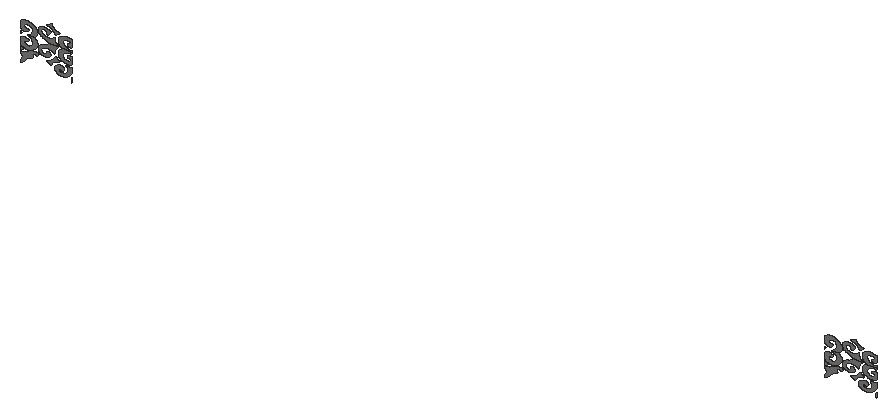
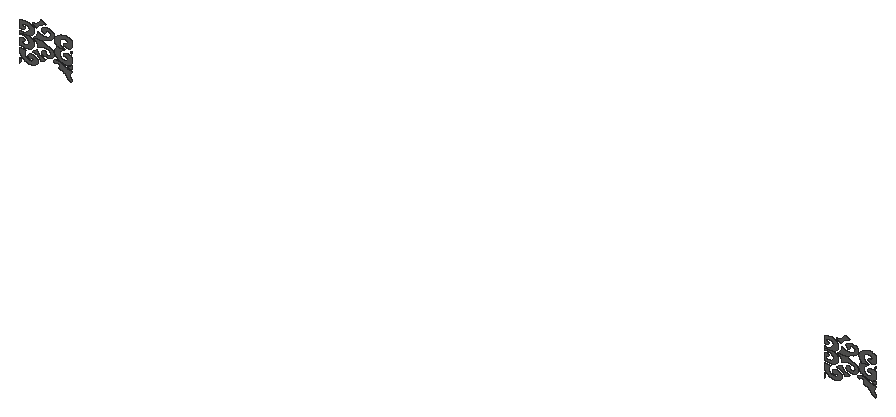
# SketchUp Ruby script. Lengths in inches.
U = 1.inch
M = Sketchup.active_model
def pt(a) = Geom::Point3d.new(a.map { |v| v * U })
def face(e, loops, mat)
  f = e.add_face(loops[0].map { |a| pt(a) })
  loops[1..].each { |l| e.add_face(l.map { |a| pt(a) }).erase! }
  f.material = f.back_material = mat if mat
  f
end
# faces: each face lists its corners as indices into pts; further lists are holes
def faces(e, pts, list, mat = nil) = list.each { |f| face(e, (f[0].is_a?(Array) ? f : [f]).map { |l| l.map { |i| pts[i] } }, mat) }
# xy, xz, yz: faces in a plane at the given z, y or x. An outline is a flat list of corners, or four numbers for a rectangle; further outlines are holes
def ring(l) = l.size == 4 ? [[l[0], l[1]], [l[2], l[1]], [l[2], l[3]], [l[0], l[3]]] : l.each_slice(2).to_a
def flat(e, list, mat, &to3) = list.each { |f| face(e, (f[0].is_a?(Array) ? f : [f]).map { |l| ring(l).map { |u, v| to3.(u, v) } }, mat) }
def xy(e, z, list, mat = nil) = flat(e, list, mat) { |x, y| [x, y, z] }
def xz(e, y, list, mat = nil) = flat(e, list, mat) { |x, z| [x, y, z] }
def yz(e, x, list, mat = nil) = flat(e, list, mat) { |y, z| [x, y, z] }
def lines(e, pts, list) = list.each { |a, b| e.add_line(pt(pts[a]), pt(pts[b])) }
# prism: a flat outline (further loops are holes) pulled along v
def prism(e, loops, v, mat = nil)
  f = face(e, loops, mat); d = Geom::Vector3d.new(v.map { |x| x * U })
  f.pushpull(f.normal.samedirection?(d) ? d.length : -d.length)
end
def box(e, o, s, mat = nil) = prism(e, [[o, [o[0] + s[0], o[1], o[2]], [o[0] + s[0], o[1] + s[1], o[2]], [o[0], o[1] + s[1], o[2]]]], [0, 0, s[2]], mat)
def at(x, y, z, deg = 0) = Geom::Transformation.translation(pt([x, y, z])) * Geom::Transformation.rotation(ORIGIN, Z_AXIS, deg.degrees)
def axes(o, x, y, z) = Geom::Transformation.new([*x, 0, *y, 0, *z, 0, *pt(o).to_a, 1])
def part(name) = M.definitions.add(name)
# library, detail: a bought-in or finely detailed component or shape, given as its bounding box
def library(name, o, s) = part(name).tap { |d| box(d.entities, o, s) }
def detail(e, o, s) = box(e.add_group.entities, o, s)
def put(e, d, t, mat = nil) = e.add_instance(d, t).tap { |i| i.material = mat if mat }
def group(e, t, mat = nil) = e.add_group.tap { |g| g.transformation = t; g.material = mat if mat }.entities
root = M.entities
M.materials.add("[0043_SaddleBrown]4").color = [124, 123, 122]
xz(root,589.17,[[449.07,580.05,448.85,580.56,448.66,581.07,448.52,581.59,448.42,582.11,448.35,582.63,448.33,583.15,448.35,583.68,448.42,584.2,448.52,584.72,448.66,585.24,448.85,585.75,449.07,586.26],[1699.7,580.05,1699.47,580.56,1699.29,581.07,1699.14,581.59,1699.04,582.11,1698.98,582.63,1698.96,583.15,1698.98,583.68,1699.04,584.2,1699.14,584.72,1699.29,585.24,1699.47,585.75,1699.7,586.26],[368.68,580.61,368.68,583.34,369.7,584.11,370.56,584.96,371.24,585.86,371.73,586.8125,372.03,587.79,372.13,588.78,372.03,589.78,371.73,590.76,371.24,591.71,370.56,592.61,369.7,593.46,368.68,594.23,368.68,595.13,369.97,595.29,371.24,595.5,372.49,595.74,373.72,596.03,374.93,596.35,376.1,596.71,377.24,597.11,378.35,597.55,379.42,598.02,380.44,598.53,381.42,599.0625,382.36,599.63,383.09,600.07,383.86,600.47,384.69,600.83,385.55,601.16,386.45,601.46,387.375,601.71,388.33,601.92,389.3125,602.08,390.31,602.21,391.32,602.28,392.33,602.32,393.35,602.31,394.16,602.23,394.92,602.03,395.6,601.74,396.15,601.36,396.54,600.91,396.76,600.43,396.8,599.92,396.65,599.42,396.32,598.95,395.83,598.54,395.21,598.21,394.48,597.98,394.37,598.49,394.05,598.96,393.54,599.37,392.875,599.68,392.1,599.88,391.27,599.95,390.45,599.88,389.67,599.68,389.01,599.37,388.5,598.96,388.18,598.49,388.07,597.98,388.03,597.57,388,597.17,387.99,596.76,388,596.36,388.03,595.95,388.07,595.55,388.14,595.15,388.22,594.74,388.3125,594.34,388.43,593.95,388.5625,593.55,388.71,593.15,387.25,592.79,385.84,592.36,384.48,591.86,383.2,591.3,381.99,590.67,380.87,589.99,379.84,589.26,378.91,588.48,378.08,587.65,377.37,586.79,376.76,585.89,376.27,584.97,375.75,584.54,375.2,584.125,374.64,583.72,374.05,583.32,373.44,582.94,372.81,582.57,372.17,582.21,371.51,581.86,370.82,581.53,370.125,581.21,369.41,580.9],[1619.31,580.61,1619.31,583.34,1620.33,584.11,1621.18,584.96,1621.86,585.86,1622.36,586.8125,1622.66,587.79,1622.76,588.78,1622.66,589.78,1622.36,590.76,1621.86,591.71,1621.18,592.61,1620.33,593.46,1619.31,594.23,1619.31,595.13,1620.59,595.29,1621.87,595.5,1623.12,595.74,1624.35,596.03,1625.55,596.35,1626.73,596.71,1627.87,597.11,1628.97,597.55,1630.04,598.02,1631.07,598.53,1632.05,599.0625,1632.98,599.63,1633.71,600.07,1634.49,600.47,1635.31,600.83,1636.17,601.16,1637.07,601.46,1638,601.71,1638.96,601.92,1639.9375,602.08,1640.93,602.21,1641.94,602.28,1642.95,602.32,1643.97,602.31,1644.79,602.23,1645.55,602.03,1646.22,601.74,1646.77,601.36,1647.17,600.91,1647.39,600.43,1647.43,599.92,1647.28,599.42,1646.95,598.95,1646.46,598.54,1645.83,598.21,1645.1,597.98,1644.99,598.49,1644.67,598.96,1644.16,599.37,1643.5,599.68,1642.73,599.88,1641.9,599.95,1641.07,599.88,1640.3,599.68,1639.63,599.37,1639.125,598.96,1638.81,598.49,1638.7,597.98,1638.65,597.57,1638.625,597.17,1638.62,596.76,1638.63,596.36,1638.65,595.95,1638.7,595.55,1638.76,595.15,1638.84,594.74,1638.9375,594.34,1639.05,593.95,1639.1875,593.55,1639.34,593.15,1637.875,592.79,1636.46,592.36,1635.11,591.86,1633.83,591.3,1632.62,590.67,1631.5,589.99,1630.47,589.26,1629.54,588.48,1628.71,587.65,1627.99,586.79,1627.39,585.89,1626.9,584.97,1626.375,584.54,1625.83,584.125,1625.26,583.72,1624.67,583.32,1624.07,582.94,1623.44,582.57,1622.79,582.21,1622.13,581.86,1621.45,581.53,1620.75,581.21,1620.04,580.9],[432.72,583.36,431.31,583.46,429.92,583.66,428.58,583.96,426.64,584.61,424.95,585.48,423.5625,586.54,422.53,587.74,421.9,589.04,421.68,590.39,421.9,591.74,422.53,593.04,423.5625,594.24,424.95,595.29,426.64,596.16,428.58,596.82,429.22,597.05,429.91,597.21,430.64,597.31,431.38,597.33,432.12,597.28,432.84,597.17,433.52,596.98,434.14,596.73,434.68,596.42,435.15,596.0625,435.51,595.66,435.77,595.23,436.13,594.85,436.41,594.45,436.58,594.02,436.66,593.58,436.63,593.14,436.51,592.7,436.29,592.28,435.97,591.89,435.5625,591.52,435.08,591.2,434.52,590.92,433.91,590.6875,433.55,590.8,433.21,590.93,432.88,591.07,432.57,591.23,432.28,591.4,432.01,591.58,431.76,591.78,431.54,591.98,431.33,592.19,431.15,592.41,431,592.64,430.87,592.87,430.1,592.59,429.4375,592.22,428.89,591.79,428.49,591.3,428.24,590.77,428.16,590.23,428.24,589.68,428.49,589.15,428.89,588.66,429.4375,588.23,430.1,587.86,430.87,587.58,431.8,587.56,432.73,587.58,433.66,587.64,434.58,587.75,435.48,587.9,436.36,588.09,437.22,588.32,438.04,588.58,438.84,588.89,439.59,589.23,440.3,589.6,440.96,590,441.54,590.79,442.01,591.6,442.36,592.43,442.58,593.28,442.68,594.14,442.65,595,442.5,595.85,442.22,596.7,441.82,597.52,441.3,598.32,440.67,599.09,439.92,599.82,440.68,599.65,441.47,599.53,442.26,599.46,443.07,599.42,443.87,599.43,444.67,599.48,445.47,599.57,446.24,599.7,447,599.88,447.72,600.09,448.42,600.35,449.07,600.64,449.07,593.03,448.71,592.48,448.33,591.93,447.93,591.39,447.52,590.85,447.1,590.3125,446.65,589.78,446.2,589.26,445.72,588.74,445.24,588.23,444.74,587.72,444.22,587.21,443.69,586.71,442.83,586.02,441.85,585.38,440.75,584.82,439.5625,584.34,438.29,583.95,436.95,583.66,435.56,583.46,434.14,583.36],
  [1683.35,583.36,1681.93,583.46,1680.54,583.66,1679.2,583.96,1677.27,584.61,1675.58,585.48,1674.1875,586.54,1673.16,587.74,1672.52,589.04,1672.31,590.39,1672.52,591.74,1673.16,593.04,1674.1875,594.24,1675.58,595.29,1677.27,596.16,1679.2,596.82,1679.85,597.05,1680.54,597.21,1681.26,597.31,1682.01,597.33,1682.75,597.28,1683.46,597.17,1684.14,596.98,1684.76,596.73,1685.31,596.42,1685.77,596.0625,1686.14,595.66,1686.39,595.23,1686.76,594.85,1687.03,594.45,1687.21,594.02,1687.28,593.58,1687.26,593.14,1687.13,592.7,1686.91,592.28,1686.59,591.89,1686.1875,591.52,1685.7,591.2,1685.15,590.92,1684.53,590.6875,1684.18,590.8,1683.84,590.93,1683.51,591.07,1683.2,591.23,1682.91,591.4,1682.64,591.58,1682.39,591.78,1682.16,591.98,1681.96,592.19,1681.78,592.41,1681.62,592.64,1681.49,592.87,1680.73,592.59,1680.0625,592.22,1679.52,591.79,1679.11,591.3,1678.87,590.77,1678.78,590.23,1678.87,589.68,1679.11,589.15,1679.52,588.66,1680.0625,588.23,1680.73,587.86,1681.49,587.58,1682.43,587.56,1683.36,587.58,1684.29,587.64,1685.2,587.75,1686.11,587.9,1686.99,588.09,1687.84,588.32,1688.67,588.58,1689.46,588.89,1690.21,589.23,1690.92,589.6,1691.58,590,1692.17,590.79,1692.64,591.6,1692.98,592.43,1693.21,593.28,1693.31,594.14,1693.28,595,1693.125,595.85,1692.85,596.7,1692.44,597.52,1691.92,598.32,1691.29,599.09,1690.55,599.82,1691.31,599.65,1692.09,599.53,1692.89,599.46,1693.69,599.42,1694.5,599.43,1695.3,599.48,1696.09,599.57,1696.87,599.7,1697.62,599.88,1698.35,600.09,1699.04,600.35,1699.7,600.64,1699.7,593.03,1699.33,592.48,1698.95,591.93,1698.56,591.39,1698.15,590.85,1697.72,590.3125,1697.28,589.78,1696.82,589.26,1696.35,588.74,1695.86,588.23,1695.36,587.72,1694.85,587.21,1694.32,586.71,1693.46,586.02,1692.48,585.38,1691.38,584.82,1690.1875,584.34,1688.91,583.95,1687.57,583.66,1686.18,583.46,1684.77,583.36],[417.2,593.19,416.65,593.51,416.09,593.83,415.53,594.14,414.95,594.45,414.36,594.75,413.77,595.04,413.17,595.32,412.56,595.6,411.9375,595.875,411.3125,596.14,410.68,596.4,410.04,596.65,411.64,597.11,413.18,597.64,414.65,598.25,416.03,598.92,417.32,599.66,418.52,600.46,419.61,601.32,420.58,602.23,421.4375,603.18,422.17,604.17,422.77,605.1875,423.24,606.23,423.77,605.83,424.3125,605.43,424.86,605.04,425.42,604.66,426.58,603.9,427.17,603.53,427.77,603.17,428.38,602.8125,429,602.46,429.63,602.12,430.27,601.78,428.6,601.54,426.99,601.2,425.44,600.75,423.98,600.2,422.63,599.56,421.39,598.83,420.3,598.02,419.34,597.15,418.55,596.22,417.92,595.24,417.47,594.23],[1667.83,593.19,1667.28,593.51,1666.72,593.83,1666.15,594.14,1665.57,594.45,1664.99,594.75,1664.4,595.04,1663.18,595.6,1662.5625,595.875,1661.9375,596.14,1661.3,596.4,1660.66,596.65,1662.26,597.11,1663.8,597.64,1665.27,598.25,1666.66,598.92,1667.95,599.66,1669.14,600.46,1670.23,601.32,1671.21,602.23,1672.0625,603.18,1672.79,604.17,1673.4,605.1875,1673.87,606.23,1674.4,605.83,1674.9375,605.43,1675.49,605.04,1676.05,604.66,1676.62,604.28,1677.2,603.9,1677.79,603.53,1678.4,603.17,1679.01,602.8125,1679.625,602.46,1680.25,602.12,1680.89,601.78,1679.23,601.54,1677.61,601.2,1676.07,600.75,1674.61,600.2,1673.25,599.56,1672.02,598.83,1670.92,598.02,1669.97,597.15,1669.18,596.22,1668.55,595.24,1668.1,594.23],[368.68,598.4,368.68,602.86,369.04,602.55,369.43,602.26,369.84,601.99,370.29,601.73,370.77,601.49,371.27,601.28,371.79,601.08,372.34,600.91,372.9,600.76,373.48,600.64,374.07,600.54,374.67,600.46,374.3,600.18,373.9,599.91,373.47,599.66,373.02,599.43,372.54,599.22,372.03,599.03,371.51,598.87,370.97,598.73,370.41,598.61,369.85,598.51,369.27,598.45],[1619.31,598.4,1619.31,602.86,1619.66,602.55,1620.05,602.26,1620.47,601.99,1620.92,601.73,1621.39,601.49,1621.9,601.28,1622.42,601.08,1622.96,600.91,1623.52,600.76,1624.1,600.64,1624.69,600.54,1625.29,600.46,1624.92,600.18,1624.53,599.91,1624.1,599.66,1623.64,599.43,1623.16,599.22,1622.66,599.03,1622.14,598.87,1621.6,598.73,1621.04,598.61,1620.47,598.51,1619.89,598.45],
  [406.65,601.54,404.66,601.66,402.75,602.02,401,602.62,399.48,603.42,398.25,604.39,397.38,605.5,396.89,606.69,396.74,607.57,396.72,608.46,396.82,609.34,397.05,610.21,397.4,611.07,397.88,611.9,398.47,612.71,399.17,613.48,399.98,614.21,400.89,614.9,401.9,615.53,402.99,616.11,404.14,616.38,405.27,616.6875,406.36,617.04,407.42,617.42,408.45,617.84,409.4375,618.3,410.38,618.79,411.28,619.31,412.125,619.86,412.92,620.4375,413.66,621.04,414.35,621.67,428.12,621.67,427.14,620.92,426.23,620.13,425.41,619.3,424.67,618.45,424.02,617.57,423.45,616.67,422.98,615.75,422.6,614.8125,422.32,613.86,422.13,612.9,422.04,611.9375,422.05,610.97,421.47,611.43,420.83,611.87,420.15,612.28,419.43,612.66,418.66,613,417.85,613.3125,417.01,613.59,416.14,613.83,415.25,614.03,414.33,614.1875,413.4,614.31,412.46,614.39,410.83,614.41,409.22,614.28,407.66,613.99,406.2,613.55,404.87,612.98,403.69,612.29,402.71,611.49,401.95,610.61,401.42,609.66,401.14,608.68,401.12,607.68,401.35,606.69,401.6,606.21,402,605.76,402.52,605.36,403.15,605.02,403.86,604.76,404.64,604.59,405.46,604.5,406.29,604.51,407.11,604.61,407.88,604.8,408.59,605.07,409.2,605.41,409.36,605.62,409.51,605.83,409.63,606.05,409.73,606.27,409.82,606.5,409.88,606.73,409.92,606.96,409.94,607.1875,409.95,607.42,409.93,607.65,409.89,607.88,409.83,608.11,409.79,608.32,409.82,608.53,409.9,608.74,410.04,608.93,410.23,609.11,410.47,609.26,410.75,609.39,411.06,609.48,411.39,609.54,411.73,609.56,412.08,609.55,412.42,609.5,413.02,609.21,413.57,608.88,414.0625,608.51,414.48,608.11,414.83,607.69,415.1,607.25,415.29,606.79,415.4,606.32,415.42,605.84,415.36,605.37,415.22,604.91,415,604.45,413.79,603.47,412.29,602.66,410.55,602.05,408.64,601.67],[1657.28,601.54,1655.28,601.66,1653.37,602.02,1651.62,602.62,1650.1,603.42,1648.88,604.39,1648,605.5,1647.51,606.69,1647.36,607.57,1647.34,608.46,1647.45,609.34,1647.68,610.21,1648.03,611.07,1648.5,611.9,1649.09,612.71,1649.8,613.48,1650.61,614.21,1651.52,614.9,1652.52,615.53,1653.61,616.11,1654.77,616.38,1655.89,616.6875,1656.99,617.04,1658.05,617.42,1659.08,617.84,1660.0625,618.3,1661,618.79,1661.9,619.31,1662.75,619.86,1663.55,620.4375,1664.29,621.04,1664.97,621.67,1678.74,621.67,1677.76,620.92,1676.86,620.13,1676.03,619.3,1675.29,618.45,1674.64,617.57,1674.08,616.67,1673.61,615.75,1673.23,614.8125,1672.95,613.86,1672.76,612.9,1672.67,611.9375,1672.67,610.97,1672.09,611.43,1671.46,611.87,1670.78,612.28,1670.05,612.66,1669.28,613,1668.48,613.3125,1667.64,613.59,1666.77,613.83,1665.875,614.03,1664.96,614.1875,1664.03,614.31,1663.08,614.39,1661.46,614.41,1659.85,614.28,1658.29,613.99,1656.83,613.55,1655.49,612.98,1654.32,612.29,1653.34,611.49,1652.58,610.61,1652.05,609.66,1651.77,608.68,1651.74,607.68,1651.97,606.69,1652.23,606.21,1652.62,605.76,1653.14,605.36,1653.77,605.02,1654.49,604.76,1655.27,604.59,1656.09,604.5,1656.92,604.51,1657.73,604.61,1658.51,604.8,1659.21,605.07,1659.83,605.41,1659.99,605.62,1660.13,605.83,1660.25,606.05,1660.36,606.27,1660.44,606.5,1660.5,606.73,1660.55,606.96,1660.57,607.1875,1660.57,607.42,1660.55,607.65,1660.51,607.88,1660.45,608.11,1660.42,608.32,1660.44,608.53,1660.52,608.74,1660.66,608.93,1660.86,609.11,1661.1,609.26,1661.375,609.39,1661.68,609.48,1662.02,609.54,1662.36,609.56,1662.7,609.55,1663.04,609.5,1663.65,609.21,1664.2,608.88,1664.6875,608.51,1665.11,608.11,1665.45,607.69,1665.72,607.25,1665.91,606.79,1666.02,606.32,1666.05,605.84,1665.99,605.37,1665.84,604.91,1665.62,604.45,1664.42,603.47,1662.91,602.66,1661.17,602.05,1659.27,601.67],[379.51,601.96,377.94,601.97,376.4,602.14,374.91,602.44,373.52,602.89,372.25,603.45,371.13,604.13,370.2,604.91,369.47,605.76,368.96,606.67,368.68,607.62,368.68,614.39,369.14,615.13,369.82,615.8,370.7,616.38,371.73,616.85,372.89,617.19,374.13,617.38,375.42,617.44,376.69,617.34,377.91,617.09,379.04,616.71,380.03,616.21,380.84,615.6,381.08,615.33,381.24,615.03,381.31,614.73,381.29,614.42,381.18,614.11,380.98,613.83,380.7,613.57,380.34,613.35,379.93,613.17,379.48,613.04,378.99,612.96,378.49,612.9375,377.82,612.91,377.17,612.8125,376.5625,612.65,376.01,612.42,375.53,612.14,375.13,611.81,374.83,611.44,374.64,611.05,374.56,610.64,374.6,610.23,374.76,609.83,375.02,609.45,375.4,608.8,375.97,608.21,376.72,607.6875,377.61,607.26,378.62,606.95,379.7,606.75,380.82,606.69,381.95,606.76,383.03,606.95,384.03,607.27,385.45,608.37,386.59,609.6,387.4,610.92,387.87,612.3,388,613.7,387.77,615.1,387.2,616.47,386.29,617.76,385.07,618.96,383.57,620.02,381.82,620.9375,379.87,621.67,390.8125,621.67,392.64,620.09,394.04,618.34,394.97,616.49,395.41,614.57,395.35,612.625,394.79,610.71,393.75,608.88,392.25,607.17,390.33,605.625,388.04,604.29,385.43,603.1875,382.57,602.36,381.07,602.08],[1630.14,601.96,1628.57,601.97,1627.02,602.14,1625.54,602.44,1624.14,602.89,1622.87,603.45,1621.76,604.13,1620.83,604.91,1620.1,605.76,1619.59,606.67,1619.31,607.62,1619.31,614.39,1619.77,615.13,1620.45,615.8,1621.32,616.38,1622.36,616.85,1623.52,617.19,1624.76,617.38,1626.04,617.44,1627.32,617.34,1628.54,617.09,1629.66,616.71,1630.65,616.21,1631.47,615.6,1631.71,615.33,1631.87,615.03,1631.93,614.73,1631.91,614.42,1631.8,614.11,1631.6,613.83,1631.32,613.57,1630.97,613.35,1630.56,613.17,1630.1,613.04,1629.61,612.96,1629.11,612.9375,1628.45,612.91,1627.8,612.8125,1627.1875,612.65,1626.63,612.42,1626.15,612.14,1625.75,611.81,1625.46,611.44,1625.27,611.05,1625.19,610.64,1625.23,610.23,1625.38,609.83,1625.64,609.45,1626.02,608.8,1626.6,608.21,1627.34,607.6875,1628.23,607.26,1629.24,606.95,1630.32,606.75,1631.45,606.69,1632.57,606.76,1633.65,606.95,1634.66,607.27,1636.08,608.37,1637.21,609.6,1638.02,610.92,1638.5,612.3,1638.62,613.7,1638.39,615.1,1637.82,616.47,1636.92,617.76,1635.7,618.96,1634.2,620.02,1632.45,620.9375,1630.49,621.67,1641.4375,621.67,1643.27,620.09,1644.66,618.34,1645.59,616.49,1646.03,614.57,1645.98,612.625,1645.42,610.71,1644.38,608.88,1642.88,607.17,1640.96,605.625,1638.66,604.29,1636.06,603.1875,1633.2,602.36,1631.69,602.08],[441.35,603.16,438.65,603.34,436.06,603.85,433.68,604.66,431.61,605.74,429.92,607.05,428.69,608.54,427.96,610.15,427.77,611.82,428.1,613.47,428.18,614.32,428.39,615.16,428.72,615.98,429.17,616.78,429.73,617.56,430.41,618.3,431.2,618.99,432.09,619.64,433.07,620.24,434.13,620.78,435.27,621.26,436.48,621.67,449.07,621.67,449.07,619.15,448.77,619.38,448.43,619.6,448.05,619.78,447.63,619.9375,447.1875,620.0625,446.73,620.15,446.25,620.21,445.76,620.23,445.28,620.22,444.8,620.17,444.33,620.09,443.88,619.97,442.8,619.61,441.77,619.2,440.78,618.75,439.85,618.26,438.99,617.73,438.18,617.15,437.45,616.55,436.79,615.91,436.2,615.25,435.7,614.5625,435.27,613.85,434.9375,613.13,434.74,612.42,434.71,611.71,434.85,610.99,435.15,610.3,435.62,609.64,436.23,609.04,436.99,608.49,437.86,608.01,438.84,607.62,439.9,607.32,441.02,607.11,442.17,607.01,443.24,607.04,444.25,607.24,445.16,607.58,445.91,608.04,446.45,608.61,446.75,609.23,446.79,609.89,446.57,610.53,446.1,611.12,445.41,611.62,444.55,612,443.55,612.24,443.31,612.22,443.0625,612.24,442.82,612.27,442.6,612.34,442.4,612.42,442.22,612.53,442.08,612.65,441.97,612.79,441.9,612.93,441.875,613.08,441.89,613.24,441.95,613.38,442.23,613.79,442.625,614.17,443.11,614.5,443.67,614.78,444.31,615,444.99,615.15,445.7,615.23,446.43,615.24,447.15,615.18,447.84,615.05,448.49,614.85,449.07,614.58,449.07,604.55,446.67,603.77,444.06,603.3],
  [1691.97,603.16,1689.27,603.34,1686.68,603.85,1684.3,604.66,1682.23,605.74,1680.55,607.05,1679.32,608.54,1678.59,610.15,1678.39,611.82,1678.73,613.47,1678.81,614.32,1679.01,615.16,1679.34,615.98,1679.79,616.78,1680.36,617.56,1681.04,618.3,1681.83,618.99,1682.71,619.64,1683.69,620.24,1684.76,620.78,1685.9,621.26,1687.11,621.67,1699.7,621.67,1699.7,619.15,1699.4,619.38,1699.05,619.6,1698.67,619.78,1698.26,619.9375,1697.8125,620.0625,1697.35,620.15,1696.875,620.21,1696.39,620.23,1695.9,620.22,1695.42,620.17,1694.95,620.09,1694.51,619.97,1693.43,619.61,1692.39,619.2,1691.41,618.75,1690.48,618.26,1689.61,617.73,1688.81,617.15,1688.07,616.55,1687.41,615.91,1686.83,615.25,1686.32,614.5625,1685.9,613.85,1685.5625,613.13,1685.36,612.42,1685.33,611.71,1685.47,610.99,1685.78,610.3,1686.24,609.64,1686.86,609.04,1687.61,608.49,1688.49,608.01,1689.46,607.62,1690.52,607.32,1691.64,607.11,1692.8,607.01,1693.86,607.04,1694.88,607.24,1695.79,607.58,1696.54,608.04,1697.08,608.61,1697.375,609.23,1697.42,609.89,1697.2,610.53,1696.73,611.12,1696.04,611.62,1695.17,612,1694.18,612.24,1693.93,612.22,1693.6875,612.24,1693.45,612.27,1693.22,612.34,1693.02,612.42,1692.85,612.53,1692.7,612.65,1692.59,612.79,1692.53,612.93,1692.5,613.08,1692.52,613.24,1692.57,613.38,1692.86,613.79,1693.25,614.17,1693.73,614.5,1694.3,614.78,1694.93,615,1695.61,615.15,1696.33,615.23,1697.05,615.24,1697.77,615.18,1698.46,615.05,1699.11,614.85,1699.7,614.58,1699.7,604.55,1697.29,603.77,1694.68,603.3],[368.68,620.2,368.68,621.67,371.08,621.67,370.77,621.66,370.46,621.62,370.16,621.5625,369.88,621.48,369.62,621.37,369.38,621.24,369.18,621.1,369,620.9375,368.87,620.76,368.76,620.58,368.7,620.39],[1619.31,620.2,1619.31,621.67,1621.71,621.67,1621.39,621.66,1621.08,621.62,1620.79,621.5625,1620.51,621.48,1620.25,621.37,1620.01,621.24,1619.8,621.1,1619.63,620.9375,1619.49,620.76,1619.39,620.58,1619.33,620.39],[368.68,621.67,371.08,621.67,370.77,621.6875,370.46,621.72,370.16,621.79,369.88,621.87,369.62,621.98,369.38,622.1,369.18,622.25,369,622.41,368.87,622.58,368.76,622.76,368.7,622.95,368.68,623.15],[379.87,621.67,390.8125,621.67,392.64,623.26,394.04,625,394.97,626.86,395.41,628.78,395.35,630.72,394.79,632.63,393.75,634.47,392.25,636.18,390.33,637.72,388.04,639.06,385.43,640.16,382.57,640.99,381.07,641.26,379.51,641.39,377.94,641.37,376.4,641.21,374.91,640.9,373.52,640.46,372.25,639.89,371.13,639.21,370.2,638.4375,369.47,637.59,368.96,636.67,368.68,635.73,368.68,628.95,369.14,628.22,369.82,627.55,370.7,626.97,371.73,626.5,372.89,626.16,374.13,625.96,375.42,625.91,376.69,626.01,377.91,626.25,379.04,626.63,380.03,627.14,380.84,627.75,381.08,628.02,381.24,628.3125,381.31,628.62,381.29,628.93,381.18,629.23,380.98,629.52,380.7,629.77,380.34,630,379.93,630.17,379.48,630.31,378.99,630.38,378.49,630.41,377.82,630.44,377.17,630.53,376.5625,630.7,376.01,630.93,375.53,631.21,375.13,631.54,374.83,631.91,374.64,632.3,374.56,632.71,374.6,633.12,374.76,633.51,375.02,633.89,375.4,634.54,375.97,635.14,376.72,635.66,377.61,636.08,378.62,636.4,379.7,636.59,380.82,636.66,381.95,636.59,383.03,636.4,384.03,636.08,385.45,634.97,386.59,633.75,387.4,632.43,387.87,631.05,388,629.64,387.77,628.24,387.2,626.875,386.29,625.58,385.07,624.39,383.57,623.32,381.82,622.41],
  [414.35,621.67,428.12,621.67,427.14,622.43,426.23,623.22,425.41,624.04,424.67,624.89,424.02,625.77,423.45,626.68,422.98,627.6,422.6,628.53,422.32,629.48,422.13,630.44,422.04,631.41,422.05,632.375,421.47,631.91,420.83,631.47,420.15,631.07,419.43,630.6875,418.66,630.34,417.85,630.03,417.01,629.76,416.14,629.52,415.25,629.32,414.33,629.16,413.4,629.04,412.46,628.96,410.83,628.9375,409.22,629.07,407.66,629.36,406.2,629.79,404.87,630.37,403.69,631.06,402.71,631.86,401.95,632.74,401.42,633.68,401.14,634.67,401.12,635.67,401.35,636.65,401.6,637.14,402,637.59,402.52,637.99,403.15,638.32,403.86,638.58,404.64,638.76,405.46,638.84,406.29,638.84,407.11,638.74,407.88,638.55,408.59,638.28,409.2,637.9375,409.36,637.73,409.51,637.51,409.63,637.29,409.73,637.07,409.82,636.85,409.88,636.62,409.92,636.39,409.94,636.16,409.95,635.93,409.93,635.7,409.89,635.47,409.83,635.24,409.79,635.03,409.82,634.82,409.9,634.61,410.04,634.42,410.23,634.24,410.47,634.09,410.75,633.96,411.06,633.87,411.39,633.81,411.73,633.78,412.08,633.79,412.42,633.84,413.02,634.14,413.57,634.47,414.0625,634.84,414.48,635.23,414.83,635.66,415.1,636.1,415.29,636.56,415.4,637.03,415.42,637.5,415.36,637.97,415.22,638.44,415,638.89,413.79,639.875,412.29,640.6875,410.55,641.29,408.64,641.67,406.65,641.8,404.66,641.6875,402.75,641.32,401,640.73,399.48,639.93,398.25,638.95,397.38,637.85,396.89,636.65,396.74,635.77,396.72,634.89,396.82,634.01,397.05,633.14,397.4,632.28,397.88,631.44,398.47,630.64,399.17,629.86,399.98,629.13,400.89,628.45,401.9,627.81,402.99,627.24,404.14,626.97,405.27,626.66,406.36,626.31,407.42,625.92,408.45,625.5,409.4375,625.05,410.38,624.56,411.28,624.04,412.125,623.49,412.92,622.91,413.66,622.3],[436.48,621.67,449.07,621.67,449.07,624.2,448.77,623.96,448.43,623.75,448.05,623.56,447.63,623.41,447.1875,623.28,446.73,623.19,446.25,623.14,445.76,623.11,445.28,623.125,444.8,623.18,444.33,623.26,443.88,623.375,442.8,623.74,441.77,624.14,440.78,624.59,439.85,625.09,438.99,625.62,438.18,626.19,437.45,626.8,436.79,627.43,436.2,628.1,435.7,628.78,435.27,629.49,434.9375,630.22,434.74,630.92,434.71,631.64,434.85,632.35,435.15,633.04,435.62,633.7,436.23,634.3125,436.99,634.86,437.86,635.33,438.84,635.73,439.9,636.03,441.02,636.23,442.17,636.34,443.24,636.3,444.25,636.11,445.16,635.77,445.91,635.3,446.45,634.74,446.75,634.11,446.79,633.46,446.57,632.82,446.1,632.23,445.41,631.73,444.55,631.35,443.55,631.11,443.31,631.125,443.0625,631.11,442.82,631.07,442.6,631.01,442.4,630.92,442.22,630.82,442.08,630.69,441.97,630.56,441.9,630.41,441.875,630.26,441.89,630.11,441.95,629.96,442.23,629.55,442.625,629.18,443.11,628.85,443.67,628.57,444.31,628.35,444.99,628.2,445.7,628.11,446.43,628.1,447.15,628.16,447.84,628.3,448.49,628.5,449.07,628.76,449.07,638.8,446.67,639.57,444.06,640.04,441.35,640.1875,438.65,640,436.06,639.5,433.68,638.6875,431.61,637.61,429.92,636.29,428.69,634.8,427.96,633.2,427.77,631.53,428.1,629.875,428.18,629.03,428.39,628.1875,428.72,627.36,429.17,626.5625,429.73,625.79,430.41,625.05,431.2,624.35,432.09,623.7,433.07,623.1,434.13,622.5625,435.27,622.09],[1619.31,621.67,1621.71,621.67,1621.39,621.6875,1621.08,621.72,1620.79,621.79,1620.51,621.87,1620.25,621.98,1620.01,622.1,1619.8,622.25,1619.63,622.41,1619.49,622.58,1619.39,622.76,1619.33,622.95,1619.31,623.15],[1630.49,621.67,1641.4375,621.67,1643.27,623.26,1644.66,625,1645.59,626.86,1646.03,628.78,1645.98,630.72,1645.42,632.63,1644.38,634.47,1642.88,636.18,1640.96,637.72,1638.66,639.06,1636.06,640.16,1633.2,640.99,1631.69,641.26,1630.14,641.39,1628.57,641.37,1627.02,641.21,1625.54,640.9,1624.14,640.46,1622.87,639.89,1621.76,639.21,1620.83,638.4375,1620.1,637.59,1619.59,636.67,1619.31,635.73,1619.31,628.95,1619.77,628.22,1620.45,627.55,1621.32,626.97,1622.36,626.5,1623.52,626.16,1624.76,625.96,1626.04,625.91,1627.32,626.01,1628.54,626.25,1629.66,626.63,1630.65,627.14,1631.47,627.75,1631.71,628.02,1631.87,628.3125,1631.93,628.62,1631.91,628.93,1631.8,629.23,1631.6,629.52,1631.32,629.77,1630.97,630,1630.56,630.17,1630.1,630.31,1629.61,630.38,1629.11,630.41,1628.45,630.44,1627.8,630.53,1627.1875,630.7,1626.63,630.93,1626.15,631.21,1625.75,631.54,1625.46,631.91,1625.27,632.3,1625.19,632.71,1625.23,633.12,1625.38,633.51,1625.64,633.89,1626.02,634.54,1626.6,635.14,1627.34,635.66,1628.23,636.08,1629.24,636.4,1630.32,636.59,1631.45,636.66,1632.57,636.59,1633.65,636.4,1634.66,636.08,1636.08,634.97,1637.21,633.75,1638.02,632.43,1638.5,631.05,1638.62,629.64,1638.39,628.24,1637.82,626.875,1636.92,625.58,1635.7,624.39,1634.2,623.32,1632.45,622.41],[1664.97,621.67,1678.74,621.67,1677.76,622.43,1676.86,623.22,1676.03,624.04,1675.29,624.89,1674.64,625.77,1674.08,626.68,1673.61,627.6,1673.23,628.53,1672.95,629.48,1672.76,630.44,1672.67,631.41,1672.67,632.375,1672.09,631.91,1671.46,631.47,1670.78,631.07,1670.05,630.6875,1669.28,630.34,1668.48,630.03,1667.64,629.76,1666.77,629.52,1665.875,629.32,1664.96,629.16,1664.03,629.04,1663.08,628.96,1661.46,628.9375,1659.85,629.07,1658.29,629.36,1656.83,629.79,1655.49,630.37,1654.32,631.06,1653.34,631.86,1652.58,632.74,1652.05,633.68,1651.77,634.67,1651.74,635.67,1651.97,636.65,1652.23,637.14,1652.62,637.59,1653.14,637.99,1653.77,638.32,1654.49,638.58,1655.27,638.76,1656.09,638.84,1656.92,638.84,1657.73,638.74,1658.51,638.55,1659.21,638.28,1659.83,637.9375,1659.99,637.73,1660.13,637.51,1660.25,637.29,1660.36,637.07,1660.44,636.85,1660.5,636.62,1660.55,636.39,1660.57,636.16,1660.57,635.93,1660.55,635.7,1660.51,635.47,1660.45,635.24,1660.42,635.03,1660.44,634.82,1660.52,634.61,1660.66,634.42,1660.86,634.24,1661.1,634.09,1661.375,633.96,1661.68,633.87,1662.02,633.81,1662.36,633.78,1662.7,633.79,1663.04,633.84,1663.65,634.14,1664.2,634.47,1664.6875,634.84,1665.11,635.23,1665.45,635.66,1665.72,636.1,1665.91,636.56,1666.02,637.03,1666.05,637.5,1665.99,637.97,1665.84,638.44,1665.62,638.89,1664.42,639.875,1662.91,640.6875,1661.17,641.29,1659.27,641.67,1657.28,641.8,1655.28,641.6875,1653.37,641.32,1651.62,640.73,1650.1,639.93,1648.88,638.95,1648,637.85,1647.51,636.65,1647.36,635.77,1647.34,634.89,1647.45,634.01,1647.68,633.14,1648.03,632.28,1648.5,631.44,1649.09,630.64,1649.8,629.86,1650.61,629.13,1651.52,628.45,1652.52,627.81,1653.61,627.24,1654.77,626.97,1655.89,626.66,1656.99,626.31,1658.05,625.92,1659.08,625.5,1660.0625,625.05,1661,624.56,1661.9,624.04,1662.75,623.49,1663.55,622.91,1664.29,622.3],
  [1687.11,621.67,1699.7,621.67,1699.7,624.2,1699.4,623.96,1699.05,623.75,1698.67,623.56,1698.26,623.41,1697.8125,623.28,1697.35,623.19,1696.875,623.14,1696.39,623.11,1695.9,623.125,1695.42,623.18,1694.95,623.26,1694.51,623.375,1693.43,623.74,1692.39,624.14,1691.41,624.59,1690.48,625.09,1689.61,625.62,1688.81,626.19,1688.07,626.8,1687.41,627.43,1686.83,628.1,1686.32,628.78,1685.9,629.49,1685.5625,630.22,1685.36,630.92,1685.33,631.64,1685.47,632.35,1685.78,633.04,1686.24,633.7,1686.86,634.3125,1687.61,634.86,1688.49,635.33,1689.46,635.73,1690.52,636.03,1691.64,636.23,1692.8,636.34,1693.86,636.3,1694.88,636.11,1695.79,635.77,1696.54,635.3,1697.08,634.74,1697.375,634.11,1697.42,633.46,1697.2,632.82,1696.73,632.23,1696.04,631.73,1695.17,631.35,1694.18,631.11,1693.93,631.125,1693.6875,631.11,1693.45,631.07,1693.22,631.01,1693.02,630.92,1692.85,630.82,1692.7,630.69,1692.59,630.56,1692.53,630.41,1692.5,630.26,1692.52,630.11,1692.57,629.96,1692.86,629.55,1693.25,629.18,1693.73,628.85,1694.3,628.57,1694.93,628.35,1695.61,628.2,1696.33,628.11,1697.05,628.1,1697.77,628.16,1698.46,628.3,1699.11,628.5,1699.7,628.76,1699.7,638.8,1697.29,639.57,1694.68,640.04,1691.97,640.1875,1689.27,640,1686.68,639.5,1684.3,638.6875,1682.23,637.61,1680.55,636.29,1679.32,634.8,1678.59,633.2,1678.39,631.53,1678.73,629.875,1678.81,629.03,1679.01,628.1875,1679.34,627.36,1679.79,626.5625,1680.36,625.79,1681.04,625.05,1681.83,624.35,1682.71,623.7,1683.69,623.1,1684.76,622.5625,1685.9,622.09],[423.24,637.11,423.77,637.51,424.3125,637.91,424.86,638.3,425.42,638.6875,426,639.07,426.58,639.44,427.17,639.8125,427.77,640.18,428.38,640.53,429,640.88,429.63,641.23,430.27,641.57,428.6,641.8,426.99,642.15,425.44,642.6,423.98,643.15,422.63,643.79,421.39,644.52,420.3,645.32,419.34,646.2,418.55,647.125,417.92,648.1,417.47,649.12,417.2,650.15,416.65,649.83,416.09,649.51,415.53,649.2,414.95,648.9,414.36,648.6,413.77,648.31,413.17,648.02,412.56,647.74,411.9375,647.47,411.3125,647.21,410.68,646.95,410.04,646.7,411.64,646.24,413.18,645.7,414.65,645.1,416.03,644.42,417.32,643.68,418.52,642.88,419.61,642.03,420.58,641.12,421.4375,640.17,422.17,639.18,422.77,638.16],[1673.87,637.11,1674.4,637.51,1674.9375,637.91,1675.49,638.3,1676.05,638.6875,1676.62,639.07,1677.2,639.44,1677.79,639.8125,1678.4,640.18,1679.01,640.53,1679.625,640.88,1680.25,641.23,1680.89,641.57,1679.23,641.8,1677.61,642.15,1676.07,642.6,1674.61,643.15,1673.25,643.79,1672.02,644.52,1670.92,645.32,1669.97,646.2,1669.18,647.125,1668.55,648.1,1668.1,649.12,1667.83,650.15,1667.28,649.83,1666.72,649.51,1666.15,649.2,1664.99,648.6,1664.4,648.31,1663.79,648.02,1663.18,647.74,1662.5625,647.47,1661.9375,647.21,1661.3,646.95,1660.66,646.7,1662.26,646.24,1663.8,645.7,1665.27,645.1,1666.66,644.42,1667.95,643.68,1669.14,642.88,1670.23,642.03,1671.21,641.12,1672.0625,640.17,1672.79,639.18,1673.4,638.16]],"[0043_SaddleBrown]4")
p = [[384.03,589.17,607.27],[384.92,589.17,607.69],[385.66,589.17,608.21],[384.03,589.17,636.08],[384.92,589.17,635.65],[385.66,589.17,635.13],
  [1634.66,589.17,607.27],[1635.55,589.17,607.69],[1636.29,589.17,608.21],[1634.66,589.17,636.08],[1635.55,589.17,635.65],[1636.29,589.17,635.13]]
lines(root,p,[[0,1],[1,2],[3,4],[4,5],[6,7],[7,8],[9,10],[10,11]])
